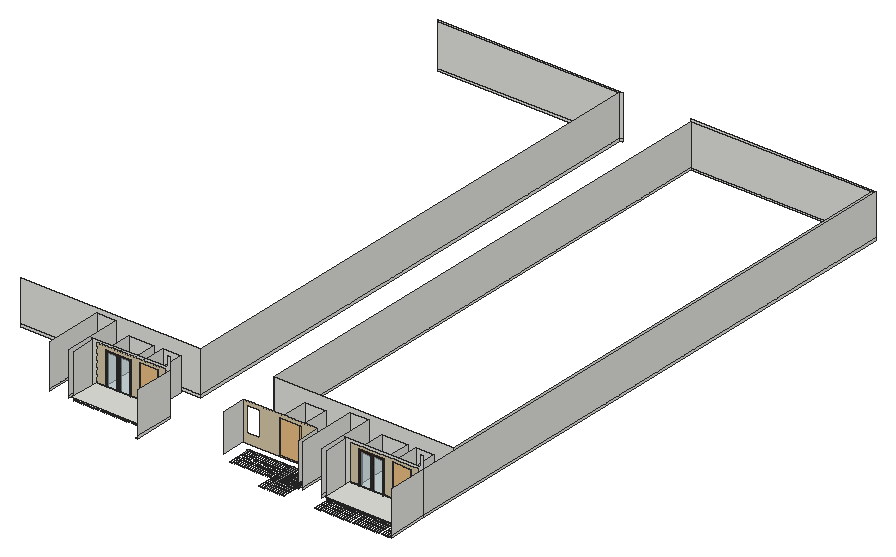
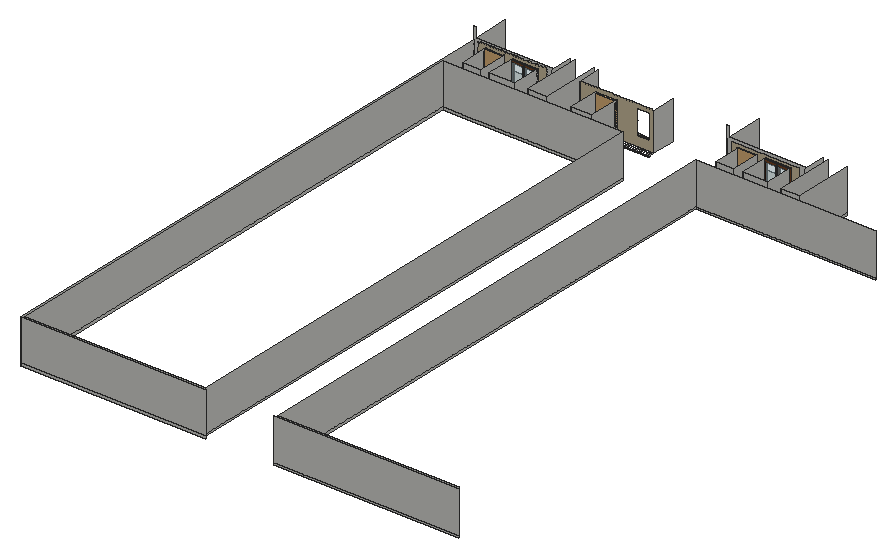
# SketchUp Ruby script. Lengths in inches.
U = 1.inch
M = Sketchup.active_model
def pt(a) = Geom::Point3d.new(a.map { |v| v * U })
def face(e, loops, mat)
  f = e.add_face(loops[0].map { |a| pt(a) })
  loops[1..].each { |l| e.add_face(l.map { |a| pt(a) }).erase! }
  f.material = f.back_material = mat if mat
  f
end
# faces: each face lists its corners as indices into pts; further lists are holes
def faces(e, pts, list, mat = nil) = list.each { |f| face(e, (f[0].is_a?(Array) ? f : [f]).map { |l| l.map { |i| pts[i] } }, mat) }
# xy, xz, yz: faces in a plane at the given z, y or x. An outline is a flat list of corners, or four numbers for a rectangle; further outlines are holes
def ring(l) = l.size == 4 ? [[l[0], l[1]], [l[2], l[1]], [l[2], l[3]], [l[0], l[3]]] : l.each_slice(2).to_a
def flat(e, list, mat, &to3) = list.each { |f| face(e, (f[0].is_a?(Array) ? f : [f]).map { |l| ring(l).map { |u, v| to3.(u, v) } }, mat) }
def xy(e, z, list, mat = nil) = flat(e, list, mat) { |x, y| [x, y, z] }
def xz(e, y, list, mat = nil) = flat(e, list, mat) { |x, z| [x, y, z] }
def yz(e, x, list, mat = nil) = flat(e, list, mat) { |y, z| [x, y, z] }
def lines(e, pts, list) = list.each { |a, b| e.add_line(pt(pts[a]), pt(pts[b])) }
# prism: a flat outline (further loops are holes) pulled along v
def prism(e, loops, v, mat = nil)
  f = face(e, loops, mat); d = Geom::Vector3d.new(v.map { |x| x * U })
  f.pushpull(f.normal.samedirection?(d) ? d.length : -d.length)
end
def box(e, o, s, mat = nil) = prism(e, [[o, [o[0] + s[0], o[1], o[2]], [o[0] + s[0], o[1] + s[1], o[2]], [o[0], o[1] + s[1], o[2]]]], [0, 0, s[2]], mat)
def at(x, y, z, deg = 0) = Geom::Transformation.translation(pt([x, y, z])) * Geom::Transformation.rotation(ORIGIN, Z_AXIS, deg.degrees)
def axes(o, x, y, z) = Geom::Transformation.new([*x, 0, *y, 0, *z, 0, *pt(o).to_a, 1])
def part(name) = M.definitions.add(name)
# library, detail: a bought-in or finely detailed component or shape, given as its bounding box
def library(name, o, s) = part(name).tap { |d| box(d.entities, o, s) }
def detail(e, o, s) = box(e.add_group.entities, o, s)
def put(e, d, t, mat = nil) = e.add_instance(d, t).tap { |i| i.material = mat if mat }
def group(e, t, mat = nil) = e.add_group.tap { |g| g.transformation = t; g.material = mat if mat }.entities
root = M.entities
M.materials.add("[Field Square Tile]").color = [216, 200, 168]
M.materials.add("[Translucent Glass Safety]").color = [204, 235, 244]
M.materials["[Translucent Glass Safety]"].alpha = 0.5
M.materials.add("[Wood Floor Parquet]").color = [140, 85, 37]
M.materials.add("[Wood Veneer 01]").color = [51, 28, 15]
M.materials.add("[Wood Veneer 01]1").color = [120, 70, 37]
c1 = library("元件\#5",[-4.39,0,0],[5.37,35.83,90.55])
c2 = part("Component\#1")
xy(c2.entities,0,[[0,0,6,48]],"[Wood Veneer 01]1")
xy(c2.entities,4,[[0,4,1.8125,44],[1.8125,4,6,44]])
xy(c2.entities,80,[[0,4,1.8125,44],[1.8125,4,6,44]])
xy(c2.entities,84,[[0,0,6,48]],"[Wood Veneer 01]1")
xz(c2.entities,0,[[0,0,6,84]],"[Wood Veneer 01]1")
xz(c2.entities,4,[[0,4,1.8125,80],[1.8125,4,6,80]])
xz(c2.entities,44,[[0,4,1.8125,80],[1.8125,4,6,80]])
xz(c2.entities,48,[[0,0,6,84]],"[Wood Veneer 01]1")
yz(c2.entities,0,[[[0,0,48,84],[4,4,44,80]]],"[Wood Veneer 01]1")
yz(c2.entities,1.8125,[[4,4,44,80]],"[Translucent Glass Safety]")
yz(c2.entities,6,[[[0,0,48,84],[4,4,44,80]]],"[Wood Veneer 01]")
c3 = part("Group\#3")
put(c3.entities,c2,at(0,0,0),"[Wood Veneer 01]")
g1 = group(c3.entities,at(0,48,0),"[Wood Veneer 01]")
xy(g1,0,[[0,0,6,48]],"[Wood Veneer 01]1")
xy(g1,4,[[0,4,1.8125,44],[1.8125,4,6,44]])
xy(g1,80,[[0,4,1.8125,44],[1.8125,4,6,44]])
xy(g1,84,[[0,0,6,48]],"[Wood Veneer 01]1")
xz(g1,0,[[0,0,6,84]],"[Wood Veneer 01]1")
xz(g1,4,[[0,4,1.8125,80],[1.8125,4,6,80]])
xz(g1,44,[[0,4,1.8125,80],[1.8125,4,6,80]])
xz(g1,48,[[0,0,6,84]],"[Wood Veneer 01]1")
yz(g1,0,[[[0,0,48,84],[4,4,44,80]]],"[Wood Veneer 01]1")
yz(g1,1.8125,[[4,4,44,80]],"[Translucent Glass Safety]")
yz(g1,6,[[[0,0,48,84],[4,4,44,80]]],"[Wood Veneer 01]")
xy(root,254.6875,[[1348.32,246.64,1350.52,361.27],[1350.52,246.64,1355.5625,361.27],[2081.89,246.64,2084.08,361.27],[2084.08,246.64,2089.125,361.27]])
xy(root,274.4375,[[1674.93,361.27,1733.6,452.64]])
xy(root,275.125,[[1142.89,273.33,1342.64,361.27],[1876.45,273.33,2076.2,361.27],[1169.05,361.27,1243.3,445.08],[1268.48,361.27,1321.23,445.08],[1902.61,361.27,1976.86,445.08],
  [2002.05,361.27,2054.8,445.08]])
xz(root,361.27,[[1723.81,253.5625,1728.56,254.6875],[1729.81,253.5625,1734.56,254.6875],[1735.81,253.5625,1740.56,254.6875],[1741.81,253.5625,1746.56,254.6875],[1747.81,253.5625,1752.56,254.6875],
  [1753.81,253.5625,1758.56,254.6875],[1759.81,253.5625,1764.56,254.6875],[1765.81,253.5625,1770.56,254.6875],[1771.81,253.5625,1776.56,254.6875],[1777.81,253.5625,1782.56,254.6875],
  [1711.81,253.875,1716.56,254.625],[1717.81,253.875,1722.56,254.6875],[1130.14,253.9375,1134.52,254.6875],[1136.14,253.9375,1140.52,254.6875],[1142.14,253.9375,1146.52,254.6875],
  [1148.14,253.9375,1152.52,254.6875],[1154.14,253.9375,1158.52,254.6875],[1160.14,253.9375,1164.52,254.6875],[1166.14,253.9375,1170.52,254.6875],[1172.14,253.9375,1176.52,254.6875],
  [1178.14,253.9375,1182.52,254.6875],[1184.14,253.9375,1188.52,254.6875],[1190.14,253.9375,1194.52,254.6875],[1196.14,253.9375,1200.52,254.6875],[1202.14,253.9375,1206.52,254.6875],
  [1208.14,253.9375,1212.52,254.6875],[1214.14,253.9375,1218.52,254.6875],[1220.14,253.9375,1224.52,254.6875],[1226.14,253.9375,1230.52,254.6875],[1232.14,253.9375,1236.52,254.6875],
  [1238.14,253.9375,1242.52,254.6875],[1244.14,253.9375,1248.52,254.6875],[1250.14,253.9375,1254.52,254.6875],[1256.14,253.9375,1260.52,254.6875],[1262.14,253.9375,1266.52,254.6875],
  [1268.14,253.9375,1272.52,254.6875],[1274.14,253.9375,1278.52,254.6875],[1280.14,253.9375,1284.52,254.6875],[1286.14,253.9375,1290.52,254.6875],[1292.14,253.9375,1296.52,254.6875],
  [1298.14,253.9375,1302.52,254.6875],[1304.14,253.9375,1308.52,254.6875],[1310.14,253.9375,1314.52,254.6875],[1316.14,253.9375,1320.52,254.6875],[1322.14,253.9375,1326.52,254.6875],
  [1328.14,253.9375,1332.52,254.6875],[1334.14,253.9375,1338.52,254.6875],[1340.14,253.9375,1344.52,254.6875],[1346.14,253.9375,1348.32,254.6875],[1579.81,253.9375,1584.56,254.6875],
  [1585.81,253.9375,1590.56,254.6875],[1591.81,253.9375,1596.56,254.6875],[1597.81,253.9375,1602.56,254.6875],[1603.81,253.9375,1608.56,254.6875],[1609.81,253.9375,1614.56,254.6875],
  [1615.81,253.9375,1620.56,254.6875],[1621.81,253.9375,1626.56,254.6875],[1627.81,253.9375,1632.56,254.6875],[1633.81,253.9375,1638.56,254.6875],[1639.81,253.9375,1644.56,254.6875],
  [1645.81,253.9375,1650.56,254.6875],[1651.81,253.9375,1656.56,254.6875],[1657.81,253.9375,1662.56,254.6875],[1663.81,253.9375,1668.56,254.6875],[1669.81,253.9375,1674.56,254.6875],
  [1675.81,253.9375,1680.56,254.6875],[1681.81,253.9375,1686.56,254.6875],[1687.81,253.9375,1692.56,254.6875],[1693.81,253.9375,1698.56,254.6875],[1699.81,253.9375,1704.56,254.6875],
  [1705.81,253.9375,1710.56,254.6875],[1863.7,253.9375,1868.08,254.6875],[1869.7,253.9375,1874.08,254.6875],[1875.7,253.9375,1880.08,254.6875],[1881.7,253.9375,1886.08,254.6875],
  [1887.7,253.9375,1892.08,254.6875],[1893.7,253.9375,1898.08,254.6875],[1899.7,253.9375,1904.08,254.6875],[1905.7,253.9375,1910.08,254.6875],[1911.7,253.9375,1916.08,254.6875],
  [1917.7,253.9375,1922.08,254.6875],[1923.7,253.9375,1928.08,254.6875],[1929.7,253.9375,1934.08,254.6875],[1935.7,253.9375,1940.08,254.6875],[1941.7,253.9375,1946.08,254.6875],
  [1947.7,253.9375,1952.08,254.6875],[1953.7,253.9375,1958.08,254.6875],[1959.7,253.9375,1964.08,254.6875],[1965.7,253.9375,1970.08,254.6875],[1971.7,253.9375,1976.08,254.6875],
  [1977.7,253.9375,1982.08,254.6875],[1983.7,253.9375,1988.08,254.6875],[1989.7,253.9375,1994.08,254.6875],[1995.7,253.9375,2000.08,254.6875],[2001.7,253.9375,2006.08,254.6875],
  [2007.7,253.9375,2012.08,254.6875],[2013.7,253.9375,2018.08,254.6875],[2019.7,253.9375,2024.08,254.6875],[2025.7,253.9375,2030.08,254.6875],[2031.7,253.9375,2036.08,254.6875],
  [2037.7,253.9375,2042.08,254.6875],[2043.7,253.9375,2048.08,254.6875],[2049.7,253.9375,2054.08,254.6875],[2055.7,253.9375,2060.08,254.6875],[2061.7,253.9375,2066.08,254.6875],
  [2067.7,253.9375,2072.08,254.6875],[2073.7,253.9375,2078.08,254.6875],[2079.7,253.9375,2081.89,254.6875],[1711.81,254.625,1716.56,254.6875],[[1130.14,254.6875,1130.14,386.6875,1348.32,386.6875,1348.32,416.75,1355.5625,416.75,1355.5625,254.6875],[1169.05,260.6875,1243.3,260.6875,1243.3,275.125,1268.48,275.125,1268.48,260.6875,1321.23,260.6875,1321.23,275.125,1342.64,275.125,1342.64,380.6875,1339.3,380.6875,1339.3,380.1875,1334.89,380.1875,1334.89,380.6875,1333.3,380.6875,1333.3,380.1875,1328.89,380.1875,1328.89,380.6875,1327.3,380.6875,1327.3,380.1875,1322.89,380.1875,1322.89,380.6875,1321.3,380.6875,1321.3,380.1875,1316.89,380.1875,1316.89,380.6875,1315.3,380.6875,1315.3,380.1875,1310.89,380.1875,1310.89,380.6875,1309.3,380.6875,1309.3,380.1875,1304.89,380.1875,1304.89,380.6875,1303.3,380.6875,1303.3,380.0625,1298.89,380.0625,1298.89,380.6875,1297.3,380.6875,1297.3,380.0625,1292.89,380.0625,1292.89,380.6875,1291.3,380.6875,1291.3,380.0625,1286.89,380.0625,1286.89,380.6875,1285.3,380.6875,1285.3,380.0625,1280.89,380.0625,1280.89,380.6875,1279.3,380.6875,1279.3,380.0625,1274.89,380.0625,1274.89,380.6875,1273.3,380.6875,1273.3,380.0625,1268.89,380.0625,1268.89,380.6875,1267.3,380.6875,1267.3,380.0625,1262.89,380.0625,1262.89,380.6875,1261.3,380.6875,1261.3,380.0625,1256.89,380.0625,1256.89,380.6875,1255.3,380.6875,1255.3,380.0625,1250.89,380.0625,1250.89,380.6875,1249.3,380.6875,1249.3,380.0625,1244.89,380.0625,1244.89,380.6875,1243.3,380.6875,1243.3,380.0625,1238.89,380.0625,1238.89,380.6875,1237.3,380.6875,1237.3,379.5625,1232.89,379.5625,1232.89,380.6875,1231.3,380.6875,1231.3,379.5625,1226.89,379.5625,1226.89,380.6875,1225.3,380.6875,1225.3,379.5625,1220.89,379.5625,1220.89,380.6875,1219.3,380.6875,1219.3,379.5625,1214.89,379.5625,1214.89,380.6875,1213.3,380.6875,1213.3,379.5625,1208.89,379.5625,1208.89,380.6875,1207.3,380.6875,1207.3,379.5625,1202.89,379.5625,1202.89,380.6875,1201.3,380.6875,1201.3,379.5625,1196.89,379.5625,1196.89,380.6875,1195.3,380.6875,1195.3,379.5625,1190.89,379.5625,1190.89,380.6875,1189.3,380.6875,1189.3,379.5625,1184.89,379.5625,1184.89,380.6875,1183.3,380.6875,1183.3,379.5625,1178.89,379.5625,1178.89,380.6875,1177.3,380.6875,1177.3,379.5625,1172.89,379.5625,1172.89,380.6875,1171.3,380.6875,1171.3,379.5625,1166.89,379.5625,1166.89,380.6875,1165.3,380.6875,1165.3,379.5625,1160.89,379.5625,1160.89,380.6875,1159.3,380.6875,1159.3,379.5625,1154.89,379.5625,1154.89,380.6875,1153.3,380.6875,1153.3,379.5625,1148.89,379.5625,1148.89,380.6875,1147.3,380.6875,1147.3,379.5625,1142.89,379.5625,1142.89,275.125,1169.05,275.125]],
  [[1863.7,254.6875,1863.7,386.6875,2081.89,386.6875,2081.89,416.75,2089.125,416.75,2089.125,254.6875],[1902.61,260.6875,1976.86,260.6875,1976.86,275.125,2002.05,275.125,2002.05,260.6875,2054.8,260.6875,2054.8,275.125,2076.2,275.125,2076.2,380.6875,2072.86,380.6875,2072.86,380.1875,2068.45,380.1875,2068.45,380.6875,2066.86,380.6875,2066.86,380.1875,2062.45,380.1875,2062.45,380.6875,2060.86,380.6875,2060.86,380.1875,2056.45,380.1875,2056.45,380.6875,2054.86,380.6875,2054.86,380.1875,2050.45,380.1875,2050.45,380.6875,2048.86,380.6875,2048.86,380.1875,2044.45,380.1875,2044.45,380.6875,2042.86,380.6875,2042.86,380.1875,2038.45,380.1875,2038.45,380.6875,2036.86,380.6875,2036.86,380.0625,2032.45,380.0625,2032.45,380.6875,2030.86,380.6875,2030.86,380.0625,2026.45,380.0625,2026.45,380.6875,2024.86,380.6875,2024.86,380.0625,2020.45,380.0625,2020.45,380.6875,2018.86,380.6875,2018.86,380.0625,2014.45,380.0625,2014.45,380.6875,2012.86,380.6875,2012.86,380.0625,2008.45,380.0625,2008.45,380.6875,2006.86,380.6875,2006.86,380.0625,2002.45,380.0625,2002.45,380.6875,2000.86,380.6875,2000.86,380.0625,1996.45,380.0625,1996.45,380.6875,1994.86,380.6875,1994.86,380.0625,1990.45,380.0625,1990.45,380.6875,1988.86,380.6875,1988.86,380.0625,1984.45,380.0625,1984.45,380.6875,1982.86,380.6875,1982.86,380.0625,1978.45,380.0625,1978.45,380.6875,1976.86,380.6875,1976.86,380.0625,1972.45,380.0625,1972.45,380.6875,1970.86,380.6875,1970.86,379.5625,1966.45,379.5625,1966.45,380.6875,1964.86,380.6875,1964.86,379.5625,1960.45,379.5625,1960.45,380.6875,1958.86,380.6875,1958.86,379.5625,1954.45,379.5625,1954.45,380.6875,1952.86,380.6875,1952.86,379.5625,1948.45,379.5625,1948.45,380.6875,1946.86,380.6875,1946.86,379.5625,1942.45,379.5625,1942.45,380.6875,1940.86,380.6875,1940.86,379.5625,1936.45,379.5625,1936.45,380.6875,1934.86,380.6875,1934.86,379.5625,1930.45,379.5625,1930.45,380.6875,1928.86,380.6875,1928.86,379.5625,1924.45,379.5625,1924.45,380.6875,1922.86,380.6875,1922.86,379.5625,1918.45,379.5625,1918.45,380.6875,1916.86,380.6875,1916.86,379.5625,1912.45,379.5625,1912.45,380.6875,1910.86,380.6875,1910.86,379.5625,1906.45,379.5625,1906.45,380.6875,1904.86,380.6875,1904.86,379.5625,1900.45,379.5625,1900.45,380.6875,1898.86,380.6875,1898.86,379.5625,1894.45,379.5625,1894.45,380.6875,1892.86,380.6875,1892.86,379.5625,1888.45,379.5625,1888.45,380.6875,1886.86,380.6875,1886.86,379.5625,1882.45,379.5625,1882.45,380.6875,1880.86,380.6875,1880.86,379.5625,1876.45,379.5625,1876.45,275.125,1902.61,275.125]],[1169.05,260.6875,1243.3,275.125],[1268.48,260.6875,1321.23,275.125],[1902.61,260.6875,1976.86,275.125],[2002.05,260.6875,2054.8,275.125]])
xz(root,361.27,[[[1567.3,269.0625,1782.56,269.0625,1782.56,378.875,1777.52,378.875,1777.52,380.6875,1774.15,380.6875,1774.15,378.875,1769.11,378.875,1769.11,380.6875,1765.73,380.6875,1765.73,378.875,1760.7,378.875,1760.7,380.6875,1757.32,380.6875,1757.32,378.875,1752.28,378.875,1752.28,380.6875,1748.91,380.6875,1748.91,378.875,1743.87,378.875,1743.87,380.6875,1740.5,380.6875,1740.5,378.875,1735.46,378.875,1735.46,380.6875,1732.08,380.6875,1732.08,378.875,1727.05,378.875,1727.05,380.6875,1723.67,380.6875,1723.67,378.875,1718.63,378.875,1718.63,380.6875,1715.26,380.6875,1715.26,378.875,1710.22,378.875,1710.22,380.6875,1706.85,380.6875,1706.85,378.875,1701.81,378.875,1701.81,380.6875,1698.43,380.6875,1698.43,378.875,1693.39,378.875,1693.39,380.6875,1690.02,380.6875,1690.02,378.875,1684.98,378.875,1684.98,380.6875,1681.61,380.6875,1681.61,378.875,1676.57,378.875,1676.57,380.6875,1673.19,380.6875,1673.19,378.875,1668.16,378.875,1668.16,380.6875,1664.78,380.6875,1664.78,378.875,1659.74,378.875,1659.74,380.6875,1656.37,380.6875,1656.37,378.875,1651.33,378.875,1651.33,380.6875,1647.96,380.6875,1647.96,378.875,1642.92,378.875,1642.92,380.6875,1639.54,380.6875,1639.54,378.875,1634.51,378.875,1634.51,380.6875,1631.13,380.6875,1631.13,378.875,1626.09,378.875,1626.09,380.6875,1622.72,380.6875,1622.72,378.875,1617.68,378.875,1617.68,380.6875,1614.3,380.6875,1614.3,378.875,1609.27,378.875,1609.27,380.6875,1605.89,380.6875,1605.89,378.875,1600.85,378.875,1600.85,380.6875,1597.48,380.6875,1597.48,378.875,1592.44,378.875,1592.44,380.6875,1589.07,380.6875,1589.07,378.875,1584.03,378.875,1584.03,380.6875,1580.65,380.6875,1580.65,378.875,1575.62,378.875,1575.62,380.6875,1572.24,380.6875,1572.24,378.875,1567.3,378.875],[1674.93,274.4375,1733.6,369.36],[1579.05,297.24,1616.36,369.37]],[1142.89,275.125,1169.05,275.125,1169.05,369.625,1243.3,369.625,1243.3,275.125,1268.48,275.125,1268.48,369.6875,1321.23,369.6875,1321.23,275.125,1342.64,275.125,1342.64,380.6875,1339.3,380.6875,1339.3,380.1875,1334.89,380.1875,1334.89,380.6875,1333.3,380.6875,1333.3,380.1875,1328.89,380.1875,1328.89,380.6875,1327.3,380.6875,1327.3,380.1875,1322.89,380.1875,1322.89,380.6875,1321.3,380.6875,1321.3,380.1875,1316.89,380.1875,1316.89,380.6875,1315.3,380.6875,1315.3,380.1875,1310.89,380.1875,1310.89,380.6875,1309.3,380.6875,1309.3,380.1875,1304.89,380.1875,1304.89,380.6875,1303.3,380.6875,1303.3,380.0625,1298.89,380.0625,1298.89,380.6875,1297.3,380.6875,1297.3,380.0625,1292.89,380.0625,1292.89,380.6875,1291.3,380.6875,1291.3,380.0625,1286.89,380.0625,1286.89,380.6875,1285.3,380.6875,1285.3,380.0625,1280.89,380.0625,1280.89,380.6875,1279.3,380.6875,1279.3,380.0625,1274.89,380.0625,1274.89,380.6875,1273.3,380.6875,1273.3,380.0625,1268.89,380.0625,1268.89,380.6875,1267.3,380.6875,1267.3,380.0625,1262.89,380.0625,1262.89,380.6875,1261.3,380.6875,1261.3,380.0625,1256.89,380.0625,1256.89,380.6875,1255.3,380.6875,1255.3,380.0625,1250.89,380.0625,1250.89,380.6875,1249.3,380.6875,1249.3,380.0625,1244.89,380.0625,1244.89,380.6875,1243.3,380.6875,1243.3,380.0625,1238.89,380.0625,1238.89,380.6875,1237.3,380.6875,1237.3,379.5625,1232.89,379.5625,1232.89,380.6875,1231.3,380.6875,1231.3,379.5625,1226.89,379.5625,1226.89,380.6875,1225.3,380.6875,1225.3,379.5625,1220.89,379.5625,1220.89,380.6875,1219.3,380.6875,1219.3,379.5625,1214.89,379.5625,1214.89,380.6875,1213.3,380.6875,1213.3,379.5625,1208.89,379.5625,1208.89,380.6875,1207.3,380.6875,1207.3,379.5625,1202.89,379.5625,1202.89,380.6875,1201.3,380.6875,1201.3,379.5625,1196.89,379.5625,1196.89,380.6875,1195.3,380.6875,1195.3,379.5625,1190.89,379.5625,1190.89,380.6875,1189.3,380.6875,1189.3,379.5625,1184.89,379.5625,1184.89,380.6875,1183.3,380.6875,1183.3,379.5625,1178.89,379.5625,1178.89,380.6875,1177.3,380.6875,1177.3,379.5625,1172.89,379.5625,1172.89,380.6875,1171.3,380.6875,1171.3,379.5625,1166.89,379.5625,1166.89,380.6875,1165.3,380.6875,1165.3,379.5625,1160.89,379.5625,1160.89,380.6875,1159.3,380.6875,1159.3,379.5625,1154.89,379.5625,1154.89,380.6875,1153.3,380.6875,1153.3,379.5625,1148.89,379.5625,1148.89,380.6875,1147.3,380.6875,1147.3,379.5625,1142.89,379.5625],[1876.45,275.125,1902.61,275.125,1902.61,369.625,1976.86,369.625,1976.86,275.125,2002.05,275.125,2002.05,369.6875,2054.8,369.6875,2054.8,275.125,2076.2,275.125,2076.2,380.6875,2072.86,380.6875,2072.86,380.1875,2068.45,380.1875,2068.45,380.6875,2066.86,380.6875,2066.86,380.1875,2062.45,380.1875,2062.45,380.6875,2060.86,380.6875,2060.86,380.1875,2056.45,380.1875,2056.45,380.6875,2054.86,380.6875,2054.86,380.1875,2050.45,380.1875,2050.45,380.6875,2048.86,380.6875,2048.86,380.1875,2044.45,380.1875,2044.45,380.6875,2042.86,380.6875,2042.86,380.1875,2038.45,380.1875,2038.45,380.6875,2036.86,380.6875,2036.86,380.0625,2032.45,380.0625,2032.45,380.6875,2030.86,380.6875,2030.86,380.0625,2026.45,380.0625,2026.45,380.6875,2024.86,380.6875,2024.86,380.0625,2020.45,380.0625,2020.45,380.6875,2018.86,380.6875,2018.86,380.0625,2014.45,380.0625,2014.45,380.6875,2012.86,380.6875,2012.86,380.0625,2008.45,380.0625,2008.45,380.6875,2006.86,380.6875,2006.86,380.0625,2002.45,380.0625,2002.45,380.6875,2000.86,380.6875,2000.86,380.0625,1996.45,380.0625,1996.45,380.6875,1994.86,380.6875,1994.86,380.0625,1990.45,380.0625,1990.45,380.6875,1988.86,380.6875,1988.86,380.0625,1984.45,380.0625,1984.45,380.6875,1982.86,380.6875,1982.86,380.0625,1978.45,380.0625,1978.45,380.6875,1976.86,380.6875,1976.86,380.0625,1972.45,380.0625,1972.45,380.6875,1970.86,380.6875,1970.86,379.5625,1966.45,379.5625,1966.45,380.6875,1964.86,380.6875,1964.86,379.5625,1960.45,379.5625,1960.45,380.6875,1958.86,380.6875,1958.86,379.5625,1954.45,379.5625,1954.45,380.6875,1952.86,380.6875,1952.86,379.5625,1948.45,379.5625,1948.45,380.6875,1946.86,380.6875,1946.86,379.5625,1942.45,379.5625,1942.45,380.6875,1940.86,380.6875,1940.86,379.5625,1936.45,379.5625,1936.45,380.6875,1934.86,380.6875,1934.86,379.5625,1930.45,379.5625,1930.45,380.6875,1928.86,380.6875,1928.86,379.5625,1924.45,379.5625,1924.45,380.6875,1922.86,380.6875,1922.86,379.5625,1918.45,379.5625,1918.45,380.6875,1916.86,380.6875,1916.86,379.5625,1912.45,379.5625,1912.45,380.6875,1910.86,380.6875,1910.86,379.5625,1906.45,379.5625,1906.45,380.6875,1904.86,380.6875,1904.86,379.5625,1900.45,379.5625,1900.45,380.6875,1898.86,380.6875,1898.86,379.5625,1894.45,379.5625,1894.45,380.6875,1892.86,380.6875,1892.86,379.5625,1888.45,379.5625,1888.45,380.6875,1886.86,380.6875,1886.86,379.5625,1882.45,379.5625,1882.45,380.6875,1880.86,380.6875,1880.86,379.5625,1876.45,379.5625]],"[Field Square Tile]")
xz(root,445.08,[[1169.05,275.125,1243.3,369.625],[1268.48,275.125,1321.23,369.6875],[1902.61,275.125,1976.86,369.625],[2002.05,275.125,2054.8,369.6875]])
xz(root,452.64,[[1674.93,274.4375,1733.6,369.36]])
xz(root,465.02,[[1061.59,254.6875,1116.3,260.6875],[1795.15,254.6875,1849.87,260.6875],[1061.59,260.6875,1116.3,380.6875],[1795.15,260.6875,1849.87,380.6875]])
xz(root,483.79,[[823.93,254.6875,1348.32,260.6875],[1557.49,254.6875,2081.89,260.6875],[823.93,260.6875,1348.32,380.6875],[1557.49,260.6875,2081.89,380.6875]])
xz(root,1996.66,[[823.93,254.6875,1348.32,260.6875],[1557.49,254.6875,2081.89,260.6875],[823.93,260.6875,1348.32,380.6875],[1557.49,260.6875,2081.89,380.6875]])
xz(root,2003.89,[[816.6875,254.6875,1355.5625,260.6875],[1550.25,254.6875,2089.125,260.6875],[816.6875,260.6875,1355.5625,380.6875],[1550.25,260.6875,2089.125,380.6875]])
yz(root,1061.59,[[293.45,254.6875,465.02,260.6875],[293.45,260.6875,465.02,380.6875]])
yz(root,1116.3,[[293.45,254.6875,465.02,260.6875],[293.45,260.6875,465.02,380.6875]])
yz(root,1130.14,[[293.45,253.9375,361.27,254.6875],[293.45,254.6875,361.27,260.6875],[293.45,260.6875,361.27,380.6875]])
yz(root,1136.14,[[293.45,253.9375,361.27,254.6875]])
yz(root,1142.14,[[293.45,253.9375,361.27,254.6875]])
yz(root,1148.14,[[293.45,253.9375,361.27,254.6875]])
yz(root,1154.14,[[293.45,253.9375,361.27,254.6875]])
yz(root,1160.14,[[293.45,253.9375,361.27,254.6875]])
yz(root,1166.14,[[293.45,253.9375,361.27,254.6875]])
yz(root,1169.05,[[361.27,275.125,445.08,369.625]])
yz(root,1172.14,[[293.45,253.9375,361.27,254.6875]])
yz(root,1178.14,[[293.45,253.9375,361.27,254.6875]])
yz(root,1184.14,[[293.45,253.9375,361.27,254.6875]])
yz(root,1190.14,[[293.45,253.9375,361.27,254.6875]])
yz(root,1196.14,[[293.45,253.9375,361.27,254.6875]])
yz(root,1202.14,[[293.45,253.9375,361.27,254.6875]])
yz(root,1208.14,[[293.45,253.9375,361.27,254.6875]])
yz(root,1214.14,[[293.45,253.9375,361.27,254.6875]])
yz(root,1220.14,[[293.45,253.9375,361.27,254.6875]])
yz(root,1226.14,[[293.45,253.9375,361.27,254.6875]])
yz(root,1232.14,[[293.45,253.9375,361.27,254.6875]])
yz(root,1238.14,[[293.45,253.9375,361.27,254.6875]])
yz(root,1243.3,[[361.27,275.125,445.08,369.625]])
yz(root,1244.14,[[293.45,253.9375,361.27,254.6875]])
yz(root,1250.14,[[293.45,253.9375,361.27,254.6875]])
yz(root,1256.14,[[293.45,253.9375,361.27,254.6875]])
yz(root,1262.14,[[293.45,253.9375,361.27,254.6875]])
yz(root,1268.14,[[293.45,253.9375,361.27,254.6875]])
yz(root,1268.48,[[361.27,275.125,445.08,369.6875]])
yz(root,1274.14,[[293.45,253.9375,361.27,254.6875]])
yz(root,1280.14,[[293.45,253.9375,361.27,254.6875]])
yz(root,1286.14,[[293.45,253.9375,361.27,254.6875]])
yz(root,1292.14,[[293.45,253.9375,361.27,254.6875]])
yz(root,1298.14,[[293.45,253.9375,361.27,254.6875]])
yz(root,1304.14,[[293.45,253.9375,361.27,254.6875]])
yz(root,1310.14,[[293.45,253.9375,361.27,254.6875]])
yz(root,1316.14,[[293.45,253.9375,361.27,254.6875]])
yz(root,1321.23,[[361.27,275.125,445.08,369.6875]])
yz(root,1322.14,[[293.45,253.9375,361.27,254.6875]])
yz(root,1328.14,[[293.45,253.9375,361.27,254.6875]])
yz(root,1334.14,[[293.45,253.9375,361.27,254.6875]])
yz(root,1340.14,[[293.45,253.9375,361.27,254.6875]])
yz(root,1346.14,[[293.45,253.9375,361.27,254.6875]])
yz(root,1348.32,[[246.64,253.9375,361.27,254.6875],[483.79,254.6875,1996.66,260.6875],[483.79,260.6875,1996.66,380.6875]])
yz(root,1355.5625,[[246.64,254.6875,361.27,260.6875],[246.64,260.6875,361.27,380.6875]])
yz(root,1557.49,[[483.79,254.6875,1996.66,260.6875],[483.79,260.6875,1996.66,380.6875]])
yz(root,1567.3,[[293.46,269.0625,361.27,378.875]])
yz(root,1584.56,[[293.45,253.9375,361.27,254.6875]])
yz(root,1590.56,[[293.45,253.9375,361.27,254.6875]])
yz(root,1596.56,[[293.45,253.9375,361.27,254.6875]])
yz(root,1602.56,[[293.45,253.9375,361.27,254.6875]])
yz(root,1608.56,[[293.45,253.9375,361.27,254.6875]])
yz(root,1614.56,[[293.45,253.9375,361.27,254.6875]])
yz(root,1620.56,[[293.45,253.9375,361.27,254.6875]])
yz(root,1626.56,[[293.45,253.9375,361.27,254.6875]])
yz(root,1632.56,[[293.45,253.9375,361.27,254.6875]])
yz(root,1638.56,[[293.45,253.9375,361.27,254.6875]])
yz(root,1644.56,[[293.45,253.9375,361.27,254.6875]])
yz(root,1650.56,[[293.45,253.9375,361.27,254.6875]])
yz(root,1656.56,[[293.45,253.9375,361.27,254.6875]])
yz(root,1662.56,[[293.45,253.9375,361.27,254.6875]])
yz(root,1668.56,[[293.45,253.9375,361.27,254.6875]])
yz(root,1674.56,[[293.45,253.9375,361.27,254.6875]])
yz(root,1674.93,[[361.27,274.4375,452.64,369.36]])
yz(root,1680.56,[[293.45,253.9375,361.27,254.6875]])
yz(root,1686.56,[[293.45,253.9375,361.27,254.6875]])
yz(root,1692.56,[[293.45,253.9375,361.27,254.6875]])
yz(root,1698.56,[[293.45,253.9375,361.27,254.6875]])
yz(root,1704.56,[[293.45,253.9375,361.27,254.6875]])
yz(root,1705.81,[[246.64,253.9375,361.27,254.6875]])
yz(root,1710.56,[[293.45,253.9375,361.27,254.6875]])
yz(root,1711.81,[[246.64,253.875,361.27,254.625],[246.64,254.625,361.27,254.6875]])
yz(root,1716.56,[[293.45,253.875,361.27,254.625],[293.45,254.625,361.27,254.6875]])
yz(root,1717.81,[[246.64,253.875,361.27,254.6875]])
yz(root,1722.56,[[293.45,253.875,361.27,254.6875]])
yz(root,1723.81,[[246.64,253.5625,361.27,254.6875]])
yz(root,1728.56,[[293.45,253.5625,361.27,254.6875]])
yz(root,1729.81,[[246.64,253.5625,361.27,254.6875]])
yz(root,1733.6,[[361.27,274.4375,452.64,369.36]])
yz(root,1734.56,[[293.45,253.5625,361.27,254.6875]])
yz(root,1735.81,[[246.64,253.5625,361.27,254.6875]])
yz(root,1740.56,[[293.45,253.5625,361.27,254.6875]])
yz(root,1741.81,[[246.64,253.5625,361.27,254.6875]])
yz(root,1746.56,[[293.45,253.5625,361.27,254.6875]])
yz(root,1747.81,[[246.64,253.5625,361.27,254.6875]])
yz(root,1752.56,[[293.45,253.5625,361.27,254.6875]])
yz(root,1753.81,[[246.64,253.5625,361.27,254.6875]])
yz(root,1758.56,[[293.45,253.5625,361.27,254.6875]])
yz(root,1759.81,[[246.64,253.5625,361.27,254.6875]])
yz(root,1764.56,[[293.45,253.5625,361.27,254.6875]])
yz(root,1765.81,[[246.64,253.5625,361.27,254.6875]])
yz(root,1770.56,[[293.45,253.5625,361.27,254.6875]])
yz(root,1771.81,[[246.64,253.5625,361.27,254.6875]])
yz(root,1776.56,[[293.45,253.5625,361.27,254.6875]])
yz(root,1777.81,[[246.64,253.5625,361.27,254.6875]])
yz(root,1782.56,[[293.45,253.5625,361.27,254.6875],[293.45,269.0625,361.27,378.875]])
yz(root,1795.15,[[293.45,254.6875,465.02,260.6875],[293.45,260.6875,465.02,380.6875]])
yz(root,1849.87,[[293.45,254.6875,465.02,260.6875],[293.45,260.6875,465.02,380.6875]])
yz(root,1863.7,[[293.45,253.9375,361.27,254.6875],[293.45,254.6875,361.27,260.6875],[293.45,260.6875,361.27,380.6875]])
yz(root,1868.08,[[246.64,253.9375,361.27,254.6875]])
yz(root,1869.7,[[293.45,253.9375,361.27,254.6875]])
yz(root,1874.08,[[246.64,253.9375,361.27,254.6875]])
yz(root,1875.7,[[293.45,253.9375,361.27,254.6875]])
yz(root,1880.08,[[246.64,253.9375,361.27,254.6875]])
yz(root,1881.7,[[293.45,253.9375,361.27,254.6875]])
yz(root,1886.08,[[246.64,253.9375,361.27,254.6875]])
yz(root,1887.7,[[293.45,253.9375,361.27,254.6875]])
yz(root,1892.08,[[246.64,253.9375,361.27,254.6875]])
yz(root,1893.7,[[293.45,253.9375,361.27,254.6875]])
yz(root,1898.08,[[246.64,253.9375,361.27,254.6875]])
yz(root,1899.7,[[293.45,253.9375,361.27,254.6875]])
yz(root,1902.61,[[361.27,275.125,445.08,369.625]])
yz(root,1904.08,[[246.64,253.9375,361.27,254.6875]])
yz(root,1905.7,[[293.45,253.9375,361.27,254.6875]])
yz(root,1910.08,[[246.64,253.9375,361.27,254.6875]])
yz(root,1911.7,[[293.45,253.9375,361.27,254.6875]])
yz(root,1916.08,[[246.64,253.9375,361.27,254.6875]])
yz(root,1917.7,[[293.45,253.9375,361.27,254.6875]])
yz(root,1922.08,[[246.64,253.9375,361.27,254.6875]])
yz(root,1923.7,[[293.45,253.9375,361.27,254.6875]])
yz(root,1928.08,[[246.64,253.9375,361.27,254.6875]])
yz(root,1929.7,[[293.45,253.9375,361.27,254.6875]])
yz(root,1934.08,[[246.64,253.9375,361.27,254.6875]])
yz(root,1935.7,[[293.45,253.9375,361.27,254.6875]])
yz(root,1940.08,[[246.64,253.9375,361.27,254.6875]])
yz(root,1941.7,[[293.45,253.9375,361.27,254.6875]])
yz(root,1946.08,[[246.64,253.9375,361.27,254.6875]])
yz(root,1947.7,[[293.45,253.9375,361.27,254.6875]])
yz(root,1952.08,[[246.64,253.9375,361.27,254.6875]])
yz(root,1953.7,[[293.45,253.9375,361.27,254.6875]])
yz(root,1958.08,[[246.64,253.9375,361.27,254.6875]])
yz(root,1959.7,[[293.45,253.9375,361.27,254.6875]])
yz(root,1964.08,[[246.64,253.9375,361.27,254.6875]])
yz(root,1965.7,[[293.45,253.9375,361.27,254.6875]])
yz(root,1970.08,[[246.64,253.9375,361.27,254.6875]])
yz(root,1971.7,[[293.45,253.9375,361.27,254.6875]])
yz(root,1976.08,[[246.64,253.9375,361.27,254.6875]])
yz(root,1976.86,[[361.27,275.125,445.08,369.625]])
yz(root,1977.7,[[293.45,253.9375,361.27,254.6875]])
yz(root,1982.08,[[246.64,253.9375,361.27,254.6875]])
yz(root,1983.7,[[293.45,253.9375,361.27,254.6875]])
yz(root,1988.08,[[246.64,253.9375,361.27,254.6875]])
yz(root,1989.7,[[293.45,253.9375,361.27,254.6875]])
yz(root,1994.08,[[246.64,253.9375,361.27,254.6875]])
yz(root,1995.7,[[293.45,253.9375,361.27,254.6875]])
yz(root,2000.08,[[246.64,253.9375,361.27,254.6875]])
yz(root,2001.7,[[293.45,253.9375,361.27,254.6875]])
yz(root,2002.05,[[361.27,275.125,445.08,369.6875]])
yz(root,2006.08,[[246.64,253.9375,361.27,254.6875]])
yz(root,2007.7,[[293.45,253.9375,361.27,254.6875]])
yz(root,2012.08,[[246.64,253.9375,361.27,254.6875]])
yz(root,2013.7,[[293.45,253.9375,361.27,254.6875]])
yz(root,2018.08,[[246.64,253.9375,361.27,254.6875]])
yz(root,2019.7,[[293.45,253.9375,361.27,254.6875]])
yz(root,2024.08,[[246.64,253.9375,361.27,254.6875]])
yz(root,2025.7,[[293.45,253.9375,361.27,254.6875]])
yz(root,2030.08,[[246.64,253.9375,361.27,254.6875]])
yz(root,2031.7,[[293.45,253.9375,361.27,254.6875]])
yz(root,2036.08,[[246.64,253.9375,361.27,254.6875]])
yz(root,2037.7,[[293.45,253.9375,361.27,254.6875]])
yz(root,2042.08,[[246.64,253.9375,361.27,254.6875]])
yz(root,2043.7,[[293.45,253.9375,361.27,254.6875]])
yz(root,2048.08,[[246.64,253.9375,361.27,254.6875]])
yz(root,2049.7,[[293.45,253.9375,361.27,254.6875]])
yz(root,2054.08,[[246.64,253.9375,361.27,254.6875]])
yz(root,2054.8,[[361.27,275.125,445.08,369.6875]])
yz(root,2055.7,[[293.45,253.9375,361.27,254.6875]])
yz(root,2060.08,[[246.64,253.9375,361.27,254.6875]])
yz(root,2061.7,[[293.45,253.9375,361.27,254.6875]])
yz(root,2066.08,[[246.64,253.9375,361.27,254.6875]])
yz(root,2067.7,[[293.45,253.9375,361.27,254.6875]])
yz(root,2072.08,[[246.64,253.9375,361.27,254.6875]])
yz(root,2073.7,[[293.45,253.9375,361.27,254.6875]])
yz(root,2078.08,[[246.64,253.9375,361.27,254.6875]])
yz(root,2079.7,[[293.45,253.9375,361.27,254.6875]])
yz(root,2081.89,[[246.64,253.9375,361.27,254.6875],[483.79,254.6875,1996.66,260.6875],[483.79,260.6875,1996.66,380.6875]])
yz(root,2089.125,[[246.64,254.6875,361.27,260.6875],[361.27,254.6875,2003.89,260.6875],[246.64,260.6875,361.27,380.6875],[361.27,260.6875,2003.89,380.6875]])
put(root,c1,axes([1674.93,361.64,274.4375],[0,-1,0],[1.63746,0,0],[0,0,1.04827]))
put(root,c1,axes([1269.02,362.12,260.6875],[0,-0.89,0],[1.45734,0,0],[0,0,1.20374]),"[Wood Floor Parquet]")
put(root,c1,axes([2002.58,362.12,260.6875],[0,-0.89,0],[1.45734,0,0],[0,0,1.20374]),"[Wood Floor Parquet]")
put(root,c3,axes([1169.05,367.27,260.6875],[0,-1,0],[0.77344,0,0],[0,0,1.29687]))
put(root,c3,axes([1902.61,367.27,260.6875],[0,-1,0],[0.77344,0,0],[0,0,1.29687]))
